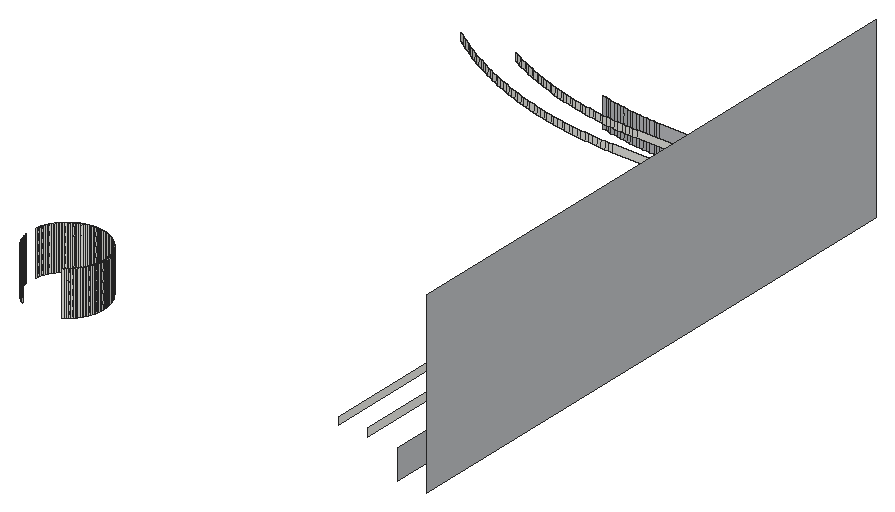
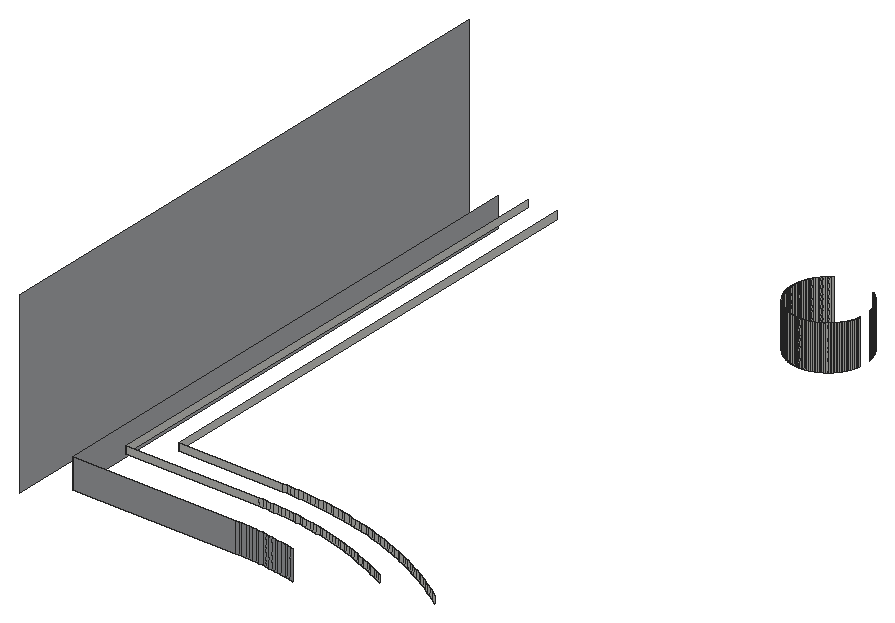
# SketchUp Ruby script. Lengths in inches.
U = 1.inch
M = Sketchup.active_model
def pt(a) = Geom::Point3d.new(a.map { |v| v * U })
def face(e, loops, mat)
  f = e.add_face(loops[0].map { |a| pt(a) })
  loops[1..].each { |l| e.add_face(l.map { |a| pt(a) }).erase! }
  f.material = f.back_material = mat if mat
  f
end
# faces: each face lists its corners as indices into pts; further lists are holes
def faces(e, pts, list, mat = nil) = list.each { |f| face(e, (f[0].is_a?(Array) ? f : [f]).map { |l| l.map { |i| pts[i] } }, mat) }
# xy, xz, yz: faces in a plane at the given z, y or x. An outline is a flat list of corners, or four numbers for a rectangle; further outlines are holes
def ring(l) = l.size == 4 ? [[l[0], l[1]], [l[2], l[1]], [l[2], l[3]], [l[0], l[3]]] : l.each_slice(2).to_a
def flat(e, list, mat, &to3) = list.each { |f| face(e, (f[0].is_a?(Array) ? f : [f]).map { |l| ring(l).map { |u, v| to3.(u, v) } }, mat) }
def xy(e, z, list, mat = nil) = flat(e, list, mat) { |x, y| [x, y, z] }
def xz(e, y, list, mat = nil) = flat(e, list, mat) { |x, z| [x, y, z] }
def yz(e, x, list, mat = nil) = flat(e, list, mat) { |y, z| [x, y, z] }
def lines(e, pts, list) = list.each { |a, b| e.add_line(pt(pts[a]), pt(pts[b])) }
# prism: a flat outline (further loops are holes) pulled along v
def prism(e, loops, v, mat = nil)
  f = face(e, loops, mat); d = Geom::Vector3d.new(v.map { |x| x * U })
  f.pushpull(f.normal.samedirection?(d) ? d.length : -d.length)
end
def box(e, o, s, mat = nil) = prism(e, [[o, [o[0] + s[0], o[1], o[2]], [o[0] + s[0], o[1] + s[1], o[2]], [o[0], o[1] + s[1], o[2]]]], [0, 0, s[2]], mat)
def at(x, y, z, deg = 0) = Geom::Transformation.translation(pt([x, y, z])) * Geom::Transformation.rotation(ORIGIN, Z_AXIS, deg.degrees)
def axes(o, x, y, z) = Geom::Transformation.new([*x, 0, *y, 0, *z, 0, *pt(o).to_a, 1])
def part(name) = M.definitions.add(name)
# library, detail: a bought-in or finely detailed component or shape, given as its bounding box
def library(name, o, s) = part(name).tap { |d| box(d.entities, o, s) }
def detail(e, o, s) = box(e.add_group.entities, o, s)
def put(e, d, t, mat = nil) = e.add_instance(d, t).tap { |i| i.material = mat if mat }
def group(e, t, mat = nil) = e.add_group.tap { |g| g.transformation = t; g.material = mat if mat }.entities
root = M.entities
M.materials.add("1427 AP 686 ARMOUR-N").color = [184, 186, 189]
xz(root,158.42,[[138.84,242,138.92,245],[138.92,242,139,245],[139,242,139.08,245],[139.08,242,139.16,245]])
xz(root,186,[[151.71,242,151.95,242.5],[151.95,242,159,242.5]])
xz(root,188,[[151.73,242,151.96,242.5],[151.96,242,161,242.5]])
xz(root,188.01,[[151.2,242,151.47,242.5]])
xz(root,190,[[151.76,240,151.97,242],[151.97,240,163,242]],"1427 AP 686 ARMOUR-N")
xz(root,190.01,[[151.28,240,151.52,242]],"1427 AP 686 ARMOUR-N")
yz(root,141.5,[[155.77,242,155.85,245],[155.85,242,155.92,245],[155.92,242,156,245],[156,242,156.08,245]])
yz(root,159,[[153.94,242,186,242.5]])
yz(root,161,[[153.9375,242,188,242.5]])
yz(root,163,[[153.93,240,190,242]],"1427 AP 686 ARMOUR-N")
yz(root,165,[[153.92,240,192,252]],"1427 AP 686 ARMOUR-N")
p = [[150.55,190.05,240],[150.79,190.04,240],[150.79,190.04,242],[150.55,190.05,242],[151.03,190.02,240],[151.03,190.02,242],
  [151.28,190.01,240],[151.28,190.01,242],[151.52,190.01,240],[151.76,190,240],[151.76,190,242],[151.52,190.01,242],
  [149.35,190.18,240],[149.59,190.15,240],[149.59,190.15,242],[149.35,190.18,242],[149.83,190.12,240],[149.83,190.12,242],
  [150.07,190.09,240],[150.07,190.09,242],[150.31,190.07,240],[150.31,190.07,242],[148.63,190.29,240],[148.87,190.25,240],
  [148.87,190.25,242],[148.63,190.29,242],[149.11,190.21,240],[149.11,190.21,242],[148.16,190.37,240],[148.39,190.33,240],
  [148.39,190.33,242],[148.16,190.37,242],[147.68,190.47,240],[147.92,190.42,240],[147.92,190.42,242],[147.68,190.47,242],
  [137.66,153.8125,242],[137.59,153.86,242],[137.59,153.86,245],[137.66,153.8125,245],[140.41,153.86,242],[140.34,153.8125,242],
  [140.34,153.8125,245],[140.41,153.86,245],[137.47,153.95,242],[137.41,154,242],[137.41,154,245],[137.47,153.95,245],
  [137.53,153.9,242],[137.53,153.9,245],[140.47,153.9,242],[140.47,153.9,245],[140.53,153.95,242],[140.53,153.95,245],
  [140.59,154,242],[140.59,154,245],[137.35,154.05,242],[137.29,154.1,242],[137.29,154.1,245],[137.35,154.05,245],
  [140.65,154.05,242],[140.65,154.05,245],[140.71,154.1,242],[140.71,154.1,245],[137.23,154.16,242],[137.23,154.16,245],
  [140.77,154.16,242],[140.77,154.16,245],[137.18,154.21,242],[137.125,154.27,242],[137.125,154.27,245],[137.18,154.21,245],
  [140.82,154.21,242],[140.82,154.21,245],[140.875,154.27,242],[140.875,154.27,245],[137.07,154.33,242],[137.02,154.39,242],
  [137.02,154.39,245],[137.07,154.33,245],[140.93,154.33,242],[140.93,154.33,245],[140.98,154.39,242],[140.98,154.39,245],
  [136.98,154.45,242],[136.98,154.45,245],[141.02,154.45,242],[141.02,154.45,245],[136.93,154.52,242],[136.89,154.58,242],
  [136.89,154.58,245],[136.93,154.52,245],[141.07,154.52,242],[141.07,154.52,245],[141.11,154.58,242],[141.11,154.58,245],
  [136.85,154.65,242],[136.85,154.65,245],[141.15,154.65,242],[141.15,154.65,245],[136.81,154.72,242],[136.77,154.79,242],
  [136.77,154.79,245],[136.81,154.72,245],[141.19,154.72,242],[141.19,154.72,245],[141.23,154.79,242],[141.23,154.79,245],
  [136.74,154.86,242],[136.74,154.86,245],[141.26,154.86,242],[141.26,154.86,245],[136.71,154.93,242],[136.68,155,242],
  [136.68,155,245],[136.71,154.93,245],[141.29,154.93,242],[141.29,154.93,245],[141.32,155,242],[141.32,155,245],
  [136.65,155.08,242],[136.65,155.08,245],[141.35,155.08,242],[141.35,155.08,245],[136.62,155.15,242],[136.62,155.15,245],
  [141.38,155.15,242],[141.38,155.15,245],[136.6,155.23,242],[136.58,155.3,242],[136.58,155.3,245],[136.6,155.23,245],
  [141.4,155.23,242],[141.4,155.23,245],[141.42,155.3,242],[141.42,155.3,245],[136.56,155.38,242],[136.56,155.38,245],
  [141.44,155.38,242],[141.44,155.38,245],[136.54,155.46,242],[136.54,155.46,245],[141.46,155.46,242],[141.46,155.46,245],
  [136.53,155.53,242],[136.53,155.53,245],[141.47,155.53,242],[141.47,155.53,245],[141.48,155.61,242],[141.48,155.61,245],
  [141.49,155.6875,242],[141.49,155.6875,245],[141.5,155.77,242],[141.5,155.77,245],[141.49,156.16,242],[141.5,156.08,242],
  [141.5,156.08,245],[141.49,156.16,245],[141.47,156.32,242],[141.48,156.24,242],[141.48,156.24,245],[141.47,156.32,245],
  [136.53,156.32,242],[136.54,156.39,242],[136.54,156.39,245],[136.53,156.32,245],[141.46,156.39,242],[141.46,156.39,245],
  [136.56,156.47,242],[136.56,156.47,245],[141.44,156.47,242],[141.44,156.47,245],[136.58,156.55,242],[136.58,156.55,245],
  [136.6,156.62,242],[136.6,156.62,245],[141.4,156.62,242],[141.42,156.55,242],[141.42,156.55,245],[141.4,156.62,245],
  [136.62,156.7,242],[136.62,156.7,245],[141.38,156.7,242],[141.38,156.7,245],[136.65,156.77,242],[136.65,156.77,245],
  [141.35,156.77,242],[141.35,156.77,245],[136.68,156.84,242],[136.68,156.84,245],[136.71,156.92,242],[136.71,156.92,245],
  [141.29,156.92,242],[141.32,156.84,242],[141.32,156.84,245],[141.29,156.92,245],[136.74,156.99,242],[136.74,156.99,245],
  [141.26,156.99,242],[141.26,156.99,245],[136.77,157.06,242],[136.77,157.06,245],[141.23,157.06,242],[141.23,157.06,245],
  [136.81,157.13,242],[136.81,157.13,245],[136.85,157.2,242],[136.85,157.2,245],[141.15,157.2,242],[141.19,157.13,242],
  [141.19,157.13,245],[141.15,157.2,245],[136.89,157.26,242],[136.89,157.26,245],[141.11,157.26,242],[141.11,157.26,245],
  [136.93,157.33,242],[136.93,157.33,245],[136.98,157.39,242],[136.98,157.39,245],[141.02,157.39,242],[141.07,157.33,242],
  [141.07,157.33,245],[141.02,157.39,245],[137.02,157.46,242],[137.02,157.46,245],[140.98,157.46,242],[140.98,157.46,245],
  [137.07,157.52,242],[137.07,157.52,245],[137.125,157.58,242],[137.125,157.58,245],[140.875,157.58,242],[140.93,157.52,242],
  [140.93,157.52,245],[140.875,157.58,245],[137.18,157.64,242],[137.18,157.64,245],[137.23,157.69,242],[137.23,157.69,245],
  [140.77,157.69,242],[140.82,157.64,242],[140.82,157.64,245],[140.77,157.69,245],[137.29,157.75,242],[137.29,157.75,245],
  [137.35,157.8,242],[137.35,157.8,245],[140.65,157.8,242],[140.71,157.75,242],[140.71,157.75,245],[140.65,157.8,245],
  [137.41,157.85,242],[137.41,157.85,245],[140.59,157.85,242],[140.59,157.85,245],[137.47,157.9,242],[137.47,157.9,245],
  [137.53,157.95,242],[137.53,157.95,245],[137.59,157.99,242],[137.59,157.99,245],[140.41,157.99,242],[140.47,157.95,242],
  [140.47,157.95,245],[140.41,157.99,245],[140.53,157.9,242],[140.53,157.9,245],[137.66,158.04,242],[137.66,158.04,245],
  [137.73,158.08,242],[137.73,158.08,245],[140.27,158.08,242],[140.34,158.04,242],[140.34,158.04,245],[140.27,158.08,245],
  [137.8,158.12,242],[137.8,158.12,245],[137.87,158.15,242],[137.87,158.15,245],[140.13,158.15,242],[140.2,158.12,242],
  [140.2,158.12,245],[140.13,158.15,245],[137.9375,158.1875,242],[137.9375,158.1875,245],[138.01,158.22,242],[138.01,158.22,245],
  [138.08,158.25,242],[138.08,158.25,245],[138.15,158.28,242],[138.15,158.28,245],[139.85,158.28,242],[139.92,158.25,242],
  [139.92,158.25,245],[139.85,158.28,245],[139.99,158.22,242],[139.99,158.22,245],[140.0625,158.1875,242],[140.0625,158.1875,245],
  [138.23,158.3,242],[138.23,158.3,245],[138.3,158.33,242],[138.3,158.33,245],[138.38,158.35,242],[138.38,158.35,245],
  [138.45,158.36,242],[138.45,158.36,245],[139.55,158.36,242],[139.62,158.35,242],[139.62,158.35,245],[139.55,158.36,245],
  [139.7,158.33,242],[139.7,158.33,245],[139.77,158.3,242],[139.77,158.3,245],[138.53,158.38,242],[138.53,158.38,245],
  [138.61,158.39,242],[138.61,158.39,245],[138.6875,158.4,242],[138.6875,158.4,245],[138.76,158.41,242],[138.76,158.41,245],
  [138.84,158.42,242],[138.84,158.42,245],[139.16,158.42,242],[139.24,158.41,242],[139.24,158.41,245],[139.16,158.42,245],
  [139.3125,158.4,242],[139.3125,158.4,245],[139.39,158.39,242],[139.39,158.39,245],[139.47,158.38,242],[139.47,158.38,245],
  [150.55,186.04,242],[150.26,186.0625,242],[150.26,186.0625,242.5],[150.55,186.04,242.5],[150.84,186.03,242],[150.84,186.03,242.5],
  [151.13,186.02,242],[151.13,186.02,242.5],[151.42,186.01,242],[151.42,186.01,242.5],[151.71,186,242],[151.71,186,242.5],
  [149.4,186.14,242],[149.11,186.17,242],[149.11,186.17,242.5],[149.4,186.14,242.5],[149.68,186.11,242],[149.68,186.11,242.5],
  [149.97,186.09,242],[149.97,186.09,242.5],[148.82,186.21,242],[148.53,186.25,242],[148.53,186.25,242.5],[148.82,186.21,242.5],
  [147.96,186.34,242],[147.67,186.39,242],[147.67,186.39,242.5],[147.96,186.34,242.5],[148.25,186.3,242],[148.25,186.3,242.5],
  [147.39,186.45,242],[147.1,186.5,242],[147.1,186.5,242.5],[147.39,186.45,242.5],[146.82,186.57,242],[146.82,186.57,242.5],
  [146.54,186.63,242],[146.26,186.7,242],[146.26,186.7,242.5],[146.54,186.63,242.5],[145.98,186.77,242],[145.98,186.77,242.5],
  [145.69,186.84,242],[145.42,186.92,242],[145.42,186.92,242.5],[145.69,186.84,242.5],[145.14,187,242],[145.14,187,242.5],
  [144.86,187.09,242],[144.86,187.09,242.5],[144.58,187.17,242],[144.58,187.17,242.5],[144.31,187.27,242],[144.31,187.27,242.5],
  [144.03,187.36,242],[144.03,187.36,242.5],[143.76,187.46,242],[143.76,187.46,242.5],[143.49,187.56,242],[143.49,187.56,242.5],
  [143.22,187.66,242],[143.22,187.66,242.5],[142.95,187.77,242],[142.95,187.77,242.5],[142.68,187.88,242],[142.68,187.88,242.5],
  [142.42,188,242],[142.42,188,242.5],[142.15,188.11,242],[142.15,188.11,242.5],[150.41,188.06,242],[150.67,188.04,242],
  [150.67,188.04,242.5],[150.41,188.06,242.5],[150.9375,188.03,242],[150.9375,188.03,242.5],[151.2,188.01,242],[151.2,188.01,242.5],
  [151.47,188.01,242],[151.73,188,242],[151.73,188,242.5],[151.47,188.01,242.5],[141.89,188.23,242],[141.89,188.23,242.5],
  [149.35,188.16,242],[149.61,188.13,242],[149.61,188.13,242.5],[149.35,188.16,242.5],[149.875,188.1,242],[149.875,188.1,242.5],
  [150.14,188.08,242],[150.14,188.08,242.5],[141.625,188.36,242],[141.625,188.36,242.5],[148.56,188.27,242],[148.82,188.23,242],
  [148.82,188.23,242.5],[148.56,188.27,242.5],[149.08,188.19,242],[149.08,188.19,242.5],[148.03,188.36,242],[148.3,188.3125,242],
  [148.3,188.3125,242.5],[148.03,188.36,242.5],[141.36,188.49,242],[141.36,188.49,242.5],[147.51,188.46,242],[147.77,188.41,242],
  [147.77,188.41,242.5],[147.51,188.46,242.5],[141.1,188.62,242],[141.1,188.62,242.5],[146.99,188.58,242],[147.25,188.52,242],
  [147.25,188.52,242.5],[146.99,188.58,242.5],[140.85,188.75,242],[140.85,188.75,242.5],[146.48,188.7,242],[146.73,188.64,242],
  [146.73,188.64,242.5],[146.48,188.7,242.5],[140.59,188.89,242],[140.59,188.89,242.5],[146.22,188.77,242],[146.22,188.77,242.5],
  [145.71,188.92,242],[145.96,188.84,242],[145.96,188.84,242.5],[145.71,188.92,242.5],[140.34,189.02,242],[140.34,189.02,242.5],
  [145.45,189,242],[145.45,189,242.5],[140.08,189.17,242],[140.08,189.17,242.5],[145.2,189.08,242],[145.2,189.08,242.5],
  [144.95,189.16,242],[144.95,189.16,242.5],[139.83,189.3125,242],[139.83,189.3125,242.5],[144.45,189.34,242],[144.7,189.25,242],
  [144.7,189.25,242.5],[144.45,189.34,242.5],[139.58,189.46,242],[139.58,189.46,242.5],[144.2,189.43,242],[144.2,189.43,242.5],
  [143.95,189.53,242],[143.95,189.53,242.5],[139.34,189.61,242],[139.34,189.61,242.5],[143.7,189.625,242],[143.7,189.625,242.5],
  [139.09,189.77,242],[139.09,189.77,242.5],[143.46,189.73,242],[143.46,189.73,242.5],[143.21,189.83,242],[143.21,189.83,242.5],
  [138.85,189.92,242],[138.85,189.92,242.5],[142.97,189.9375,242],[142.97,189.9375,242.5],[138.61,190.08,242],[138.61,190.08,242.5],
  [142.73,190.05,242],[142.73,190.05,242.5],[142.49,190.16,242],[142.49,190.16,242.5],[138.37,190.25,242],[138.37,190.25,242.5],
  [138.13,190.41,242],[138.13,190.41,242.5],[142.25,190.28,242],[142.25,190.28,242.5],[142.01,190.4,242],[142.01,190.4,242.5],
  [141.78,190.52,242],[141.78,190.52,242.5]]
faces(root,p,[[0,1,2,3],[1,4,5,2],[4,6,7,5],[8,9,10,11],[12,13,14,15],[13,16,17,14],[16,18,19,17],[18,20,21,19],
  [20,0,3,21],[22,23,24,25],[23,26,27,24],[26,12,15,27],[28,29,30,31],[29,22,25,30],[32,33,34,35],[33,28,31,34]],"1427 AP 686 ARMOUR-N")
faces(root,p,[[36,37,38,39],[40,41,42,43],[44,45,46,47],[48,44,47,49],[37,48,49,38],[50,40,43,51],[52,50,51,53],[54,52,53,55],
  [56,57,58,59],[45,56,59,46],[60,54,55,61],[62,60,61,63],[57,64,65,58],[66,62,63,67],[68,69,70,71],[64,68,71,65],
  [72,66,67,73],[74,72,73,75],[76,77,78,79],[69,76,79,70],[80,74,75,81],[82,80,81,83],[77,84,85,78],[86,82,83,87],
  [88,89,90,91],[84,88,91,85],[92,86,87,93],[94,92,93,95],[89,96,97,90],[98,94,95,99],[100,101,102,103],[96,100,103,97],
  [104,98,99,105],[106,104,105,107],[101,108,109,102],[110,106,107,111],[112,113,114,115],[108,112,115,109],[116,110,111,117],[118,116,117,119],
  [113,120,121,114],[122,118,119,123],[120,124,125,121],[126,122,123,127],[128,129,130,131],[124,128,131,125],[132,126,127,133],[134,132,133,135],
  [129,136,137,130],[138,134,135,139],[136,140,141,137],[142,138,139,143],[140,144,145,141],[146,142,143,147],[148,146,147,149],[150,148,149,151],
  [152,150,151,153],[154,155,156,157],[158,159,160,161],[159,154,157,160],[162,163,164,165],[166,158,161,167],[163,168,169,164],[170,166,167,171],
  [168,172,173,169],[172,174,175,173],[176,177,178,179],[177,170,171,178],[174,180,181,175],[182,176,179,183],[180,184,185,181],[186,182,183,187],
  [184,188,189,185],[188,190,191,189],[192,193,194,195],[193,186,187,194],[190,196,197,191],[198,192,195,199],[196,200,201,197],[202,198,199,203],
  [200,204,205,201],[204,206,207,205],[208,209,210,211],[209,202,203,210],[206,212,213,207],[214,208,211,215],[212,216,217,213],[216,218,219,217],
  [220,221,222,223],[221,214,215,222],[218,224,225,219],[226,220,223,227],[224,228,229,225],[228,230,231,229],[232,233,234,235],[233,226,227,234],
  [230,236,237,231],[236,238,239,237],[240,241,242,243],[241,232,235,242],[238,244,245,239],[244,246,247,245],[248,249,250,251],[249,240,243,250],
  [246,252,253,247],[254,248,251,255],[252,256,257,253],[256,258,259,257],[258,260,261,259],[262,263,264,265],[263,266,267,264],[266,254,255,267],
  [260,268,269,261],[268,270,271,269],[272,273,274,275],[273,262,265,274],[270,276,277,271],[276,278,279,277],[280,281,282,283],[281,272,275,282],
  [278,284,285,279],[284,286,287,285],[286,288,289,287],[288,290,291,289],[292,293,294,295],[293,296,297,294],[296,298,299,297],[298,280,283,299],
  [290,300,301,291],[300,302,303,301],[302,304,305,303],[304,306,307,305],[308,309,310,311],[309,312,313,310],[312,314,315,313],[314,292,295,315],
  [306,316,317,307],[316,318,319,317],[318,320,321,319],[320,322,323,321],[322,324,325,323],[326,327,328,329],[327,330,331,328],[330,332,333,331],
  [332,334,335,333],[334,308,311,335],[336,337,338,339],[340,336,339,341],[342,340,341,343],[344,342,343,345],[346,344,345,347],[348,349,350,351],
  [352,348,351,353],[354,352,353,355],[337,354,355,338],[356,357,358,359],[349,356,359,350],[360,361,362,363],[364,360,363,365],[357,364,365,358],
  [366,367,368,369],[361,366,369,362],[367,370,371,368],[372,373,374,375],[370,372,375,371],[373,376,377,374],[378,379,380,381],[376,378,381,377],
  [379,382,383,380],[382,384,385,383],[384,386,387,385],[386,388,389,387],[388,390,391,389],[390,392,393,391],[392,394,395,393],[394,396,397,395],
  [396,398,399,397],[398,400,401,399],[400,402,403,401],[402,404,405,403],[406,407,408,409],[407,410,411,408],[410,412,413,411],[414,415,416,417],
  [404,418,419,405],[420,421,422,423],[421,424,425,422],[424,426,427,425],[426,406,409,427],[418,428,429,419],[430,431,432,433],[431,434,435,432],
  [434,420,423,435],[436,437,438,439],[437,430,433,438],[428,440,441,429],[442,443,444,445],[443,436,439,444],[440,446,447,441],[448,449,450,451],
  [449,442,445,450],[446,452,453,447],[454,455,456,457],[455,448,451,456],[452,458,459,453],[460,454,457,461],[462,463,464,465],[463,460,461,464],
  [458,466,467,459],[468,462,465,469],[466,470,471,467],[472,468,469,473],[474,472,473,475],[470,476,477,471],[478,479,480,481],[479,474,475,480],
  [476,482,483,477],[484,478,481,485],[486,484,485,487],[482,488,489,483],[490,486,487,491],[488,492,493,489],[494,490,491,495],[496,494,495,497],
  [492,498,499,493],[500,496,497,501],[498,502,503,499],[504,500,501,505],[506,504,505,507],[502,508,509,503],[508,510,511,509],[512,506,507,513],
  [514,512,513,515],[516,514,515,517]])
